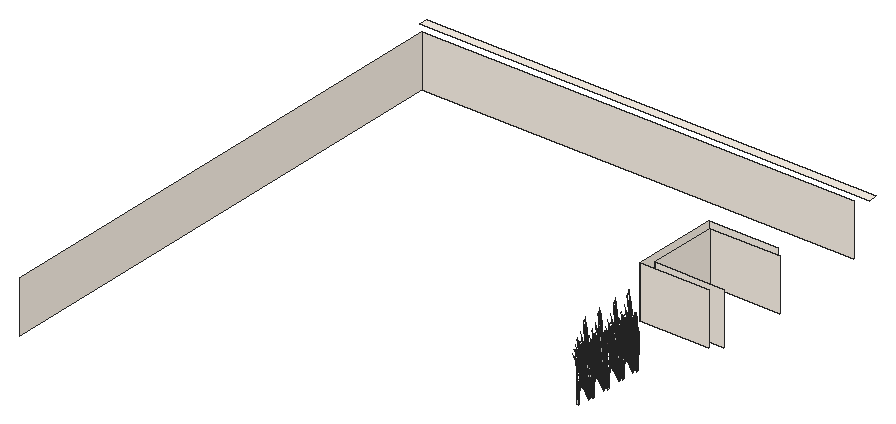
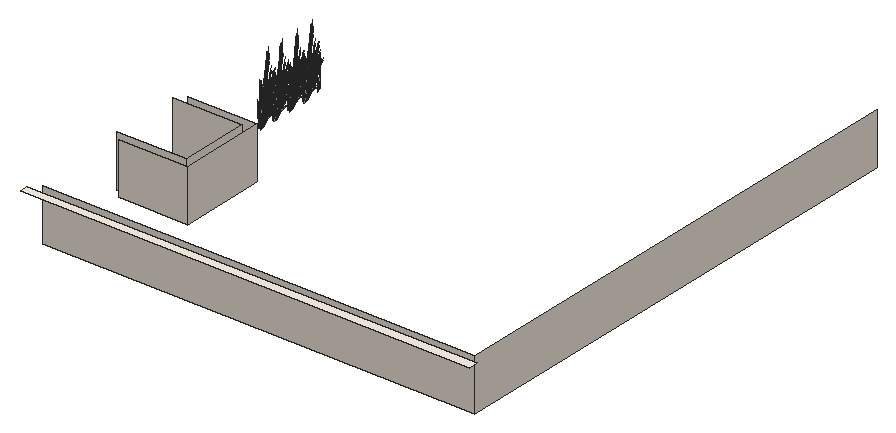
# SketchUp Ruby script. Lengths in inches.
U = 1.inch
M = Sketchup.active_model
def pt(a) = Geom::Point3d.new(a.map { |v| v * U })
def face(e, loops, mat)
  f = e.add_face(loops[0].map { |a| pt(a) })
  loops[1..].each { |l| e.add_face(l.map { |a| pt(a) }).erase! }
  f.material = f.back_material = mat if mat
  f
end
# faces: each face lists its corners as indices into pts; further lists are holes
def faces(e, pts, list, mat = nil) = list.each { |f| face(e, (f[0].is_a?(Array) ? f : [f]).map { |l| l.map { |i| pts[i] } }, mat) }
# xy, xz, yz: faces in a plane at the given z, y or x. An outline is a flat list of corners, or four numbers for a rectangle; further outlines are holes
def ring(l) = l.size == 4 ? [[l[0], l[1]], [l[2], l[1]], [l[2], l[3]], [l[0], l[3]]] : l.each_slice(2).to_a
def flat(e, list, mat, &to3) = list.each { |f| face(e, (f[0].is_a?(Array) ? f : [f]).map { |l| ring(l).map { |u, v| to3.(u, v) } }, mat) }
def xy(e, z, list, mat = nil) = flat(e, list, mat) { |x, y| [x, y, z] }
def xz(e, y, list, mat = nil) = flat(e, list, mat) { |x, z| [x, y, z] }
def yz(e, x, list, mat = nil) = flat(e, list, mat) { |y, z| [x, y, z] }
def lines(e, pts, list) = list.each { |a, b| e.add_line(pt(pts[a]), pt(pts[b])) }
# prism: a flat outline (further loops are holes) pulled along v
def prism(e, loops, v, mat = nil)
  f = face(e, loops, mat); d = Geom::Vector3d.new(v.map { |x| x * U })
  f.pushpull(f.normal.samedirection?(d) ? d.length : -d.length)
end
def box(e, o, s, mat = nil) = prism(e, [[o, [o[0] + s[0], o[1], o[2]], [o[0] + s[0], o[1] + s[1], o[2]], [o[0], o[1] + s[1], o[2]]]], [0, 0, s[2]], mat)
def at(x, y, z, deg = 0) = Geom::Transformation.translation(pt([x, y, z])) * Geom::Transformation.rotation(ORIGIN, Z_AXIS, deg.degrees)
def axes(o, x, y, z) = Geom::Transformation.new([*x, 0, *y, 0, *z, 0, *pt(o).to_a, 1])
def part(name) = M.definitions.add(name)
# library, detail: a bought-in or finely detailed component or shape, given as its bounding box
def library(name, o, s) = part(name).tap { |d| box(d.entities, o, s) }
def detail(e, o, s) = box(e.add_group.entities, o, s)
def put(e, d, t, mat = nil) = e.add_instance(d, t).tap { |i| i.material = mat if mat }
def group(e, t, mat = nil) = e.add_group.tap { |g| g.transformation = t; g.material = mat if mat }.entities
root = M.entities
M.materials.add("C01_Vanilla_Cream").color = [255, 246, 235]
M.materials.add("LightPink_Translucent").color = [144, 107, 117]
M.materials["LightPink_Translucent"].alpha = 0.75
c1 = part("blade")
p = [[2.15,0.21,22],[0,0.17,0],[0.09,0.45,0],[2.18,0.31,22],[2.29,0.31,22],[0.38,0.45,0],
  [2.48,0.24,33],[2.49,0.24,33],[2.48,0.22,33]]
faces(c1.entities,p,[[0,1,2,3],[4,5,2,3],[6,3,4,7],[8,0,3,6]])
c2 = part("seeds")
p = [[0.3,-0.1,1.38],[-0.01,-0.03,1.59],[-0.01,-0.03,0.03],[0.14,-0.07,-0.07],[0.29,-0.03,3],[0.15,0.01,3.11]]
faces(c2.entities,p,[[0,1,2,3],[1,0,4,5]],"LightPink_Translucent")
c3 = part("blade with seeds")
put(c3.entities,c1,at(0,0,0))
put(c3.entities,c2,axes([2.4,0.25,30.99],[1.5799,-0.05474,1.17369],[-0.12525,1.92788,0.29478],[-0.07173,-0.02425,1.56792]))
xy(root,690,[[48,366,360,372]],"C01_Vanilla_Cream")
xz(root,234,[[306,654,354,690]],"C01_Vanilla_Cream")
xz(root,240,[[312,654,360,690]],"C01_Vanilla_Cream")
xz(root,288,[[312,654,360,690]],"C01_Vanilla_Cream")
xz(root,294,[[306,654,354,690]],"C01_Vanilla_Cream")
xz(root,360,[[54,654,354,690]],"C01_Vanilla_Cream")
yz(root,54,[[12,654,360,690]],"C01_Vanilla_Cream")
yz(root,306,[[234,654,294,690]],"C01_Vanilla_Cream")
yz(root,312,[[240,654,288,690]],"C01_Vanilla_Cream")
put(root,c3,axes([339.83,148.68,657.18],[0.20495,-0.00938,1.40529],[-0.13596,0.40664,0.11363],[-0.29207,-0.02515,0.60075]))
put(root,c3,axes([339.83,161.3125,657.18],[0.20495,-0.00938,1.40529],[-0.13596,0.40664,0.11363],[-0.29207,-0.02515,0.60075]))
put(root,c3,axes([339.83,174.79,657.18],[0.20495,-0.00938,1.40529],[-0.13596,0.40664,0.11363],[-0.29207,-0.02515,0.60075]))
put(root,c3,axes([339.83,186.65,657.18],[0.20495,-0.00938,1.40529],[-0.13596,0.40664,0.11363],[-0.29207,-0.02515,0.60075]))
put(root,c3,axes([339.92,149.39,657.18],[0.17145,-0.08763,1.40529],[0.14434,0.4049,0.11363],[-0.26915,0.09151,0.60075]))
put(root,c3,axes([339.92,162.03,657.18],[0.17145,-0.08763,1.40529],[0.14434,0.4049,0.11363],[-0.26915,0.09151,0.60075]))
put(root,c3,axes([339.92,175.51,657.18],[0.17145,-0.08763,1.40529],[0.14434,0.4049,0.11363],[-0.26915,0.09151,0.60075]))
put(root,c3,axes([339.92,187.37,657.18],[0.17145,-0.08763,1.40529],[0.14434,0.4049,0.11363],[-0.26915,0.09151,0.60075]))
put(root,c3,axes([339.39,150.08,656.125],[0.17172,0.03401,1.17261],[0.11068,0.34736,-0.25218],[-0.23326,0.06502,0.50135]))
put(root,c3,axes([339.39,162.72,656.125],[0.17172,0.03401,1.17261],[0.11068,0.34736,-0.25218],[-0.23326,0.06502,0.50135]))
put(root,c3,axes([339.39,176.2,656.125],[0.17172,0.03401,1.17261],[0.11068,0.34736,-0.25218],[-0.23326,0.06502,0.50135]))
put(root,c3,axes([339.39,188.06,656.125],[0.17172,0.03401,1.17261],[0.11068,0.34736,-0.25218],[-0.23326,0.06502,0.50135]))
put(root,c3,axes([340.9,148.97,656.74],[0.14045,-0.05993,1.45192],[0.04843,0.41842,0.11363],[-0.30422,0.05552,0.51893]))
put(root,c3,axes([340.9,161.61,656.74],[0.14045,-0.05993,1.45192],[0.04843,0.41842,0.11363],[-0.30422,0.05552,0.51893]))
put(root,c3,axes([340.9,175.08,656.74],[0.14045,-0.05993,1.45192],[0.04843,0.41842,0.11363],[-0.30422,0.05552,0.51893]))
put(root,c3,axes([340.9,186.95,656.74],[0.14045,-0.05993,1.45192],[0.04843,0.41842,0.11363],[-0.30422,0.05552,0.51893]))
put(root,c3,axes([339.39,149.25,657.87],[-0.08069,0.05378,1.43454],[0.00686,0.39297,-0.22687],[-0.18495,0.0511,0.11505]))
put(root,c3,axes([339.39,161.89,657.87],[-0.08069,0.05378,1.43454],[0.00686,0.39297,-0.22687],[-0.18495,0.0511,0.11505]))
put(root,c3,axes([339.39,175.36,657.87],[-0.08069,0.05378,1.43454],[0.00686,0.39297,-0.22687],[-0.18495,0.0511,0.11505]))
put(root,c3,axes([339.39,187.23,657.87],[-0.08069,0.05378,1.43454],[0.00686,0.39297,-0.22687],[-0.18495,0.0511,0.11505]))
put(root,c3,axes([340.45,148.3,658.08],[-0.49394,-0.00997,-0.58257],[0.03317,-0.42002,0.0703],[-0.20925,-0.04433,0.8241]))
put(root,c3,axes([340.45,160.9375,658.08],[-0.49394,-0.00997,-0.58257],[0.03317,-0.42002,0.0703],[-0.20925,-0.04433,0.8241]))
put(root,c3,axes([340.45,174.41,658.08],[-0.49394,-0.00997,-0.58257],[0.03317,-0.42002,0.0703],[-0.20925,-0.04433,0.8241]))
put(root,c3,axes([340.45,186.27,658.08],[-0.49394,-0.00997,-0.58257],[0.03317,-0.42002,0.0703],[-0.20925,-0.04433,0.8241]))
put(root,c3,axes([340.05,148.4,656.125],[0.09647,0.11534,1.17261],[-0.2223,0.31351,-0.25218],[-0.22826,-0.07493,0.50135]))
put(root,c3,axes([340.05,161.04,656.125],[0.09647,0.11534,1.17261],[-0.2223,0.31351,-0.25218],[-0.22826,-0.07493,0.50135]))
put(root,c3,axes([340.05,174.52,656.125],[0.09647,0.11534,1.17261],[-0.2223,0.31351,-0.25218],[-0.22826,-0.07493,0.50135]))
put(root,c3,axes([340.05,186.375,656.125],[0.09647,0.11534,1.17261],[-0.2223,0.31351,-0.25218],[-0.22826,-0.07493,0.50135]))
put(root,c3,axes([339.65,149.03,657.71],[-0.41064,-0.11557,-0.29039],[0.11977,-0.33716,0.3749],[-0.16533,0.03092,0.71734]))
put(root,c3,axes([339.65,161.66,657.71],[-0.41064,-0.11557,-0.29039],[0.11977,-0.33716,0.3749],[-0.16533,0.03092,0.71734]))
put(root,c3,axes([339.65,175.14,657.71],[-0.41064,-0.11557,-0.29039],[0.11977,-0.33716,0.3749],[-0.16533,0.03092,0.71734]))
put(root,c3,axes([339.65,187,657.71],[-0.41064,-0.11557,-0.29039],[0.11977,-0.33716,0.3749],[-0.16533,0.03092,0.71734]))
put(root,c3,axes([340.22,148.02,657.18],[0.18354,0.07137,1.40529],[-0.37983,0.29943,0.11363],[-0.23673,-0.13508,0.60075]))
put(root,c3,axes([340.22,160.66,657.18],[0.18354,0.07137,1.40529],[-0.37983,0.29943,0.11363],[-0.23673,-0.13508,0.60075]))
put(root,c3,axes([340.22,174.14,657.18],[0.18354,0.07137,1.40529],[-0.37983,0.29943,0.11363],[-0.23673,-0.13508,0.60075]))
put(root,c3,axes([340.22,186,657.18],[0.18354,0.07137,1.40529],[-0.37983,0.29943,0.11363],[-0.23673,-0.13508,0.60075]))
put(root,c3,axes([338.5,149.65,657.86],[0.06306,0.01111,1.45454],[0.19508,0.36602,-0.13744],[-0.12909,0.09607,0.2574]))
put(root,c3,axes([338.5,162.28,657.86],[0.06306,0.01111,1.45454],[0.19508,0.36602,-0.13744],[-0.12909,0.09607,0.2574]))
put(root,c3,axes([338.5,175.76,657.86],[0.06306,0.01111,1.45454],[0.19508,0.36602,-0.13744],[-0.12909,0.09607,0.2574]))
put(root,c3,axes([338.5,187.625,657.86],[0.06306,0.01111,1.45454],[0.19508,0.36602,-0.13744],[-0.12909,0.09607,0.2574]))
put(root,c3,axes([339.94,149.2,657.84],[-0.13386,0.37682,-0.41901],[-0.45895,-0.12916,-0.32456],[-0.18478,0.03455,0.80174]))
put(root,c3,axes([339.94,161.84,657.84],[-0.13386,0.37682,-0.41901],[-0.45895,-0.12916,-0.32456],[-0.18478,0.03455,0.80174]))
put(root,c3,axes([339.94,175.3125,657.84],[-0.13386,0.37682,-0.41901],[-0.45895,-0.12916,-0.32456],[-0.18478,0.03455,0.80174]))
put(root,c3,axes([339.94,187.17,657.84],[-0.13386,0.37682,-0.41901],[-0.45895,-0.12916,-0.32456],[-0.18478,0.03455,0.80174]))
put(root,c3,axes([340.28,148.38,657.84],[-0.35879,0.27441,-0.41901],[-0.31422,-0.28988,-0.32456],[-0.18229,-0.04175,0.80174]))
put(root,c3,axes([340.28,161.02,657.84],[-0.35879,0.27441,-0.41901],[-0.31422,-0.28988,-0.32456],[-0.18229,-0.04175,0.80174]))
put(root,c3,axes([340.28,174.5,657.84],[-0.35879,0.27441,-0.41901],[-0.31422,-0.28988,-0.32456],[-0.18229,-0.04175,0.80174]))
put(root,c3,axes([340.28,186.36,657.84],[-0.35879,0.27441,-0.41901],[-0.31422,-0.28988,-0.32456],[-0.18229,-0.04175,0.80174]))
put(root,c3,axes([339.7,149.17,655.22],[0.01253,0.06529,1.44601],[-0.25262,0.34095,-0.2209],[-0.17944,-0.01719,0.2463]))
put(root,c3,axes([339.7,161.8125,655.22],[0.01253,0.06529,1.44601],[-0.25262,0.34095,-0.2209],[-0.17944,-0.01719,0.2463]))
put(root,c3,axes([339.7,175.29,655.22],[0.01253,0.06529,1.44601],[-0.25262,0.34095,-0.2209],[-0.17944,-0.01719,0.2463]))
put(root,c3,axes([339.7,187.15,655.22],[0.01253,0.06529,1.44601],[-0.25262,0.34095,-0.2209],[-0.17944,-0.01719,0.2463]))
put(root,c3,axes([339.78,147.61,657.86],[0.03663,0.04134,1.45454],[-0.17659,0.37163,-0.13744],[-0.17885,0.00269,0.2574]))
put(root,c3,axes([339.78,160.25,657.86],[0.03663,0.04134,1.45454],[-0.17659,0.37163,-0.13744],[-0.17885,0.00269,0.2574]))
put(root,c3,axes([339.78,173.73,657.86],[0.03663,0.04134,1.45454],[-0.17659,0.37163,-0.13744],[-0.17885,0.00269,0.2574]))
put(root,c3,axes([339.78,185.59,657.86],[0.03663,0.04134,1.45454],[-0.17659,0.37163,-0.13744],[-0.17885,0.00269,0.2574]))
put(root,c3,axes([339.03,150.81,656.27],[0.20592,-0.18775,0.94186],[0.08126,0.29723,0.69201],[-0.14881,0.05322,0.20745]))
put(root,c3,axes([339.03,163.45,656.27],[0.20592,-0.18775,0.94186],[0.08126,0.29723,0.69201],[-0.14881,0.05322,0.20745]))
put(root,c3,axes([339.03,176.92,656.27],[0.20592,-0.18775,0.94186],[0.08126,0.29723,0.69201],[-0.14881,0.05322,0.20745]))
put(root,c3,axes([339.03,188.79,656.27],[0.20592,-0.18775,0.94186],[0.08126,0.29723,0.69201],[-0.14881,0.05322,0.20745]))
put(root,c3,axes([340.1875,147.37,657.87],[-0.10632,-0.00292,1.43454],[-0.33847,0.29241,-0.22687],[-0.1806,-0.05975,0.11505]))
put(root,c3,axes([340.1875,160,657.87],[-0.10632,-0.00292,1.43454],[-0.33847,0.29241,-0.22687],[-0.1806,-0.05975,0.11505]))
put(root,c3,axes([340.1875,173.48,657.87],[-0.10632,-0.00292,1.43454],[-0.33847,0.29241,-0.22687],[-0.1806,-0.05975,0.11505]))
put(root,c3,axes([340.1875,185.34,657.87],[-0.10632,-0.00292,1.43454],[-0.33847,0.29241,-0.22687],[-0.1806,-0.05975,0.11505]))
put(root,c3,axes([339.75,148.98,657.88],[0.1396,-0.37772,0.39362],[0.45895,0.12916,0.32456],[-0.18049,0.0227,0.8145]))
put(root,c3,axes([339.75,161.62,657.88],[0.1396,-0.37772,0.39362],[0.45895,0.12916,0.32456],[-0.18049,0.0227,0.8145]))
put(root,c3,axes([339.75,175.1,657.88],[0.1396,-0.37772,0.39362],[0.45895,0.12916,0.32456],[-0.18049,0.0227,0.8145]))
put(root,c3,axes([339.75,186.96,657.88],[0.1396,-0.37772,0.39362],[0.45895,0.12916,0.32456],[-0.18049,0.0227,0.8145]))
put(root,c3,axes([339.91,148.875,658.13],[0.24861,0.37512,-0.09971],[-0.44125,0.18434,-0.55346],[-0.18594,0.04949,0.84097]))
put(root,c3,axes([339.91,161.51,658.13],[0.24861,0.37512,-0.09971],[-0.44125,0.18434,-0.55346],[-0.18594,0.04949,0.84097]))
put(root,c3,axes([339.91,174.99,658.13],[0.24861,0.37512,-0.09971],[-0.44125,0.18434,-0.55346],[-0.18594,0.04949,0.84097]))
put(root,c3,axes([339.91,186.85,658.13],[0.24861,0.37512,-0.09971],[-0.44125,0.18434,-0.55346],[-0.18594,0.04949,0.84097]))
put(root,c3,axes([340.47,148.1,658.13],[-0.02646,0.4213,-0.09971],[-0.50094,-0.01152,-0.55346],[-0.19293,-0.02926,0.84097]))
put(root,c3,axes([340.47,160.73,658.13],[-0.02646,0.4213,-0.09971],[-0.50094,-0.01152,-0.55346],[-0.19293,-0.02926,0.84097]))
put(root,c3,axes([340.47,174.21,658.13],[-0.02646,0.4213,-0.09971],[-0.50094,-0.01152,-0.55346],[-0.19293,-0.02926,0.84097]))
put(root,c3,axes([340.47,186.07,658.13],[-0.02646,0.4213,-0.09971],[-0.50094,-0.01152,-0.55346],[-0.19293,-0.02926,0.84097]))
put(root,c3,axes([340.15,148.125,657.71],[-0.28114,-0.25937,-0.29039],[0.32102,-0.24553,0.3749],[-0.16311,-0.03736,0.71734]))
put(root,c3,axes([340.15,160.76,657.71],[-0.28114,-0.25937,-0.29039],[0.32102,-0.24553,0.3749],[-0.16311,-0.03736,0.71734]))
put(root,c3,axes([340.15,174.24,657.71],[-0.28114,-0.25937,-0.29039],[0.32102,-0.24553,0.3749],[-0.16311,-0.03736,0.71734]))
put(root,c3,axes([340.15,186.1,657.71],[-0.28114,-0.25937,-0.29039],[0.32102,-0.24553,0.3749],[-0.16311,-0.03736,0.71734]))
put(root,c3,axes([339.71,148.88,657.88],[-0.18148,-0.28246,0.05273],[0.33093,-0.13825,0.41509],[-0.14588,0.02728,0.63295]))
put(root,c3,axes([339.71,161.52,657.88],[-0.18148,-0.28246,0.05273],[0.33093,-0.13825,0.41509],[-0.14588,0.02728,0.63295]))
put(root,c3,axes([339.71,175,657.88],[-0.18148,-0.28246,0.05273],[0.33093,-0.13825,0.41509],[-0.14588,0.02728,0.63295]))
put(root,c3,axes([339.71,186.86,657.88],[-0.18148,-0.28246,0.05273],[0.33093,-0.13825,0.41509],[-0.14588,0.02728,0.63295]))
put(root,c3,axes([340.55,149.66,657.18],[0.12341,-0.12729,1.40529],[0.31162,0.34357,0.11363],[-0.21373,0.15646,0.60075]))
put(root,c3,axes([340.55,162.3,657.18],[0.12341,-0.12729,1.40529],[0.31162,0.34357,0.11363],[-0.21373,0.15646,0.60075]))
put(root,c3,axes([340.55,175.78,657.18],[0.12341,-0.12729,1.40529],[0.31162,0.34357,0.11363],[-0.21373,0.15646,0.60075]))
put(root,c3,axes([340.55,187.64,657.18],[0.12341,-0.12729,1.40529],[0.31162,0.34357,0.11363],[-0.21373,0.15646,0.60075]))
put(root,c3,axes([339.8,150,657.71],[-0.43011,0.0592,-0.29039],[-0.11357,-0.33844,0.3749],[-0.12326,0.0909,0.71734]))
put(root,c3,axes([339.8,162.64,657.71],[-0.43011,0.0592,-0.29039],[-0.11357,-0.33844,0.3749],[-0.12326,0.0909,0.71734]))
put(root,c3,axes([339.8,176.11,657.71],[-0.43011,0.0592,-0.29039],[-0.11357,-0.33844,0.3749],[-0.12326,0.0909,0.71734]))
put(root,c3,axes([339.8,187.97,657.71],[-0.43011,0.0592,-0.29039],[-0.11357,-0.33844,0.3749],[-0.12326,0.0909,0.71734]))
put(root,c3,axes([339.57,151,655.22],[0.06628,0.04139,1.44601],[0.11238,0.38347,-0.2209],[-0.14689,0.08177,0.2463]))
put(root,c3,axes([339.57,163.64,655.22],[0.06628,0.04139,1.44601],[0.11238,0.38347,-0.2209],[-0.14689,0.08177,0.2463]))
put(root,c3,axes([339.57,177.12,655.22],[0.06628,0.04139,1.44601],[0.11238,0.38347,-0.2209],[-0.14689,0.08177,0.2463]))
put(root,c3,axes([339.57,188.98,655.22],[0.06628,0.04139,1.44601],[0.11238,0.38347,-0.2209],[-0.14689,0.08177,0.2463]))
put(root,c3,axes([339.47,148.75,656.27],[0.31546,-0.02964,0.94186],[-0.20011,0.26119,0.69201],[-0.15589,-0.03918,0.20745]))
put(root,c3,axes([339.47,161.38,656.27],[0.31546,-0.02964,0.94186],[-0.20011,0.26119,0.69201],[-0.15589,-0.03918,0.20745]))
put(root,c3,axes([339.47,174.86,656.27],[0.31546,-0.02964,0.94186],[-0.20011,0.26119,0.69201],[-0.15589,-0.03918,0.20745]))
put(root,c3,axes([339.47,186.72,656.27],[0.31546,-0.02964,0.94186],[-0.20011,0.26119,0.69201],[-0.15589,-0.03918,0.20745]))
put(root,c3,axes([339.86,149.92,657.88],[-0.12254,-0.38127,0.39362],[0.48071,-0.06617,0.32456],[-0.14168,0.08967,0.8145]))
put(root,c3,axes([339.86,162.5625,657.88],[-0.12254,-0.38127,0.39362],[0.48071,-0.06617,0.32456],[-0.14168,0.08967,0.8145]))
put(root,c3,axes([339.86,176.04,657.88],[-0.12254,-0.38127,0.39362],[0.48071,-0.06617,0.32456],[-0.14168,0.08967,0.8145]))
put(root,c3,axes([339.86,187.9,657.88],[-0.12254,-0.38127,0.39362],[0.48071,-0.06617,0.32456],[-0.14168,0.08967,0.8145]))
put(root,c3,axes([340.11,148.03,658.18],[0.40806,-0.30572,0.44086],[0.35193,0.32467,0.3635],[-0.19145,-0.05639,0.91224]))
put(root,c3,axes([340.11,160.67,658.18],[0.40806,-0.30572,0.44086],[0.35193,0.32467,0.3635],[-0.19145,-0.05639,0.91224]))
put(root,c3,axes([340.11,174.14,658.18],[0.40806,-0.30572,0.44086],[0.35193,0.32467,0.3635],[-0.19145,-0.05639,0.91224]))
put(root,c3,axes([340.11,186,658.18],[0.40806,-0.30572,0.44086],[0.35193,0.32467,0.3635],[-0.19145,-0.05639,0.91224]))
put(root,c3,axes([339.76,149.85,657.88],[-0.33921,-0.17422,0.05273],[0.19749,-0.2481,0.41509],[-0.10876,0.08021,0.63295]))
put(root,c3,axes([339.76,162.49,657.88],[-0.33921,-0.17422,0.05273],[0.19749,-0.2481,0.41509],[-0.10876,0.08021,0.63295]))
put(root,c3,axes([339.76,175.97,657.88],[-0.33921,-0.17422,0.05273],[0.19749,-0.2481,0.41509],[-0.10876,0.08021,0.63295]))
put(root,c3,axes([339.76,187.83,657.88],[-0.33921,-0.17422,0.05273],[0.19749,-0.2481,0.41509],[-0.10876,0.08021,0.63295]))
put(root,c3,axes([340.45,136.89,657.18],[0.092,-0.14239,1.40529],[0.38596,0.29467,0.11363],[-0.17411,0.18366,0.60075]))
put(root,c3,axes([340.45,149.98,657.18],[0.092,-0.14239,1.40529],[0.38596,0.29467,0.11363],[-0.17411,0.18366,0.60075]))
put(root,c3,axes([340.45,162.62,657.18],[0.092,-0.14239,1.40529],[0.38596,0.29467,0.11363],[-0.17411,0.18366,0.60075]))
put(root,c3,axes([340.45,176.09,657.18],[0.092,-0.14239,1.40529],[0.38596,0.29467,0.11363],[-0.17411,0.18366,0.60075]))
put(root,c3,axes([340.45,187.95,657.18],[0.092,-0.14239,1.40529],[0.38596,0.29467,0.11363],[-0.17411,0.18366,0.60075]))
put(root,c3,axes([340.09,148.99,658.14],[0.41064,0.11557,0.29039],[-0.11977,0.33716,-0.3749],[-0.16533,0.03092,0.71734]))
put(root,c3,axes([340.09,161.625,658.14],[0.41064,0.11557,0.29039],[-0.11977,0.33716,-0.3749],[-0.16533,0.03092,0.71734]))
put(root,c3,axes([340.09,175.1,658.14],[0.41064,0.11557,0.29039],[-0.11977,0.33716,-0.3749],[-0.16533,0.03092,0.71734]))
put(root,c3,axes([340.09,186.96,658.14],[0.41064,0.11557,0.29039],[-0.11977,0.33716,-0.3749],[-0.16533,0.03092,0.71734]))
put(root,c3,axes([340.16,150.04,657.84],[0.12693,0.37826,-0.41901],[-0.48071,0.06617,-0.32456],[-0.13776,0.1016,0.80174]))
put(root,c3,axes([340.16,162.67,657.84],[0.12693,0.37826,-0.41901],[-0.48071,0.06617,-0.32456],[-0.13776,0.1016,0.80174]))
put(root,c3,axes([340.16,176.15,657.84],[0.12693,0.37826,-0.41901],[-0.48071,0.06617,-0.32456],[-0.13776,0.1016,0.80174]))
put(root,c3,axes([340.16,188.01,657.84],[0.12693,0.37826,-0.41901],[-0.48071,0.06617,-0.32456],[-0.13776,0.1016,0.80174]))
put(root,c3,axes([340.29,148.03,657.88],[0.02488,-0.31501,0.05273],[0.3757,0.00864,0.41509],[-0.14392,-0.03296,0.63295]))
put(root,c3,axes([340.29,160.66,657.88],[0.02488,-0.31501,0.05273],[0.3757,0.00864,0.41509],[-0.14392,-0.03296,0.63295]))
put(root,c3,axes([340.29,174.14,657.88],[0.02488,-0.31501,0.05273],[0.3757,0.00864,0.41509],[-0.14392,-0.03296,0.63295]))
put(root,c3,axes([340.29,186,657.88],[0.02488,-0.31501,0.05273],[0.3757,0.00864,0.41509],[-0.14392,-0.03296,0.63295]))
put(root,c3,axes([339.41,137.625,657.87],[-0.01228,0.08198,1.43454],[0.34856,0.28519,-0.22687],[-0.09125,0.13486,0.11505]))
put(root,c3,axes([339.41,150.72,657.87],[-0.01228,0.08198,1.43454],[0.34856,0.28519,-0.22687],[-0.09125,0.13486,0.11505]))
put(root,c3,axes([339.41,163.35,657.87],[-0.01228,0.08198,1.43454],[0.34856,0.28519,-0.22687],[-0.09125,0.13486,0.11505]))
put(root,c3,axes([339.41,176.83,657.87],[-0.01228,0.08198,1.43454],[0.34856,0.28519,-0.22687],[-0.09125,0.13486,0.11505]))
put(root,c3,axes([339.41,188.69,657.87],[-0.01228,0.08198,1.43454],[0.34856,0.28519,-0.22687],[-0.09125,0.13486,0.11505]))
put(root,c3,axes([341.36,149.77,655.6875],[-0.514,-0.06792,-0.51129],[0.10846,-0.41895,-0.13419],[-0.15339,-0.05076,1.12859]))
put(root,c3,axes([341.36,162.4,655.6875],[-0.514,-0.06792,-0.51129],[0.10846,-0.41895,-0.13419],[-0.15339,-0.05076,1.12859]))
put(root,c3,axes([341.36,175.88,655.6875],[-0.514,-0.06792,-0.51129],[0.10846,-0.41895,-0.13419],[-0.15339,-0.05076,1.12859]))
put(root,c3,axes([341.36,187.74,655.6875],[-0.514,-0.06792,-0.51129],[0.10846,-0.41895,-0.13419],[-0.15339,-0.05076,1.12859]))
put(root,c3,axes([341.45,147.48,658.45],[-0.32977,0.39714,-0.11168],[-0.47757,-0.2288,-0.61987],[-0.16601,-0.1122,0.94188]))
put(root,c3,axes([341.45,160.12,658.45],[-0.32977,0.39714,-0.11168],[-0.47757,-0.2288,-0.61987],[-0.16601,-0.1122,0.94188]))
put(root,c3,axes([341.45,173.6,658.45],[-0.32977,0.39714,-0.11168],[-0.47757,-0.2288,-0.61987],[-0.16601,-0.1122,0.94188]))
put(root,c3,axes([341.45,185.46,658.45],[-0.32977,0.39714,-0.11168],[-0.47757,-0.2288,-0.61987],[-0.16601,-0.1122,0.94188]))
put(root,c3,axes([340.55,148.26,658.14],[0.28114,0.25937,0.29039],[-0.32102,0.24553,-0.3749],[-0.16311,-0.03736,0.71734]))
put(root,c3,axes([340.55,160.9,658.14],[0.28114,0.25937,0.29039],[-0.32102,0.24553,-0.3749],[-0.16311,-0.03736,0.71734]))
put(root,c3,axes([340.55,174.375,658.14],[0.28114,0.25937,0.29039],[-0.32102,0.24553,-0.3749],[-0.16311,-0.03736,0.71734]))
put(root,c3,axes([340.55,186.24,658.14],[0.28114,0.25937,0.29039],[-0.32102,0.24553,-0.3749],[-0.16311,-0.03736,0.71734]))
put(root,c3,axes([341.31,147.8,658.08],[-0.42133,-0.20023,-0.58257],[0.29943,-0.35088,0.0703],[-0.15265,-0.11956,0.8241]))
put(root,c3,axes([341.31,160.44,658.08],[-0.42133,-0.20023,-0.58257],[0.29943,-0.35088,0.0703],[-0.15265,-0.11956,0.8241]))
put(root,c3,axes([341.31,173.92,658.08],[-0.42133,-0.20023,-0.58257],[0.29943,-0.35088,0.0703],[-0.15265,-0.11956,0.8241]))
put(root,c3,axes([341.31,185.78,658.08],[-0.42133,-0.20023,-0.58257],[0.29943,-0.35088,0.0703],[-0.15265,-0.11956,0.8241]))
put(root,c3,axes([341.11,147.8125,657.84],[-0.48758,0.09847,-0.41901],[-0.08529,-0.37293,-0.32456],[-0.13096,-0.10687,0.80174]))
put(root,c3,axes([341.11,160.45,657.84],[-0.48758,0.09847,-0.41901],[-0.08529,-0.37293,-0.32456],[-0.13096,-0.10687,0.80174]))
put(root,c3,axes([341.11,173.93,657.84],[-0.48758,0.09847,-0.41901],[-0.08529,-0.37293,-0.32456],[-0.13096,-0.10687,0.80174]))
put(root,c3,axes([341.11,185.79,657.84],[-0.48758,0.09847,-0.41901],[-0.08529,-0.37293,-0.32456],[-0.13096,-0.10687,0.80174]))
put(root,c3,axes([340.68,150.56,655.65],[-0.46245,-0.20713,-0.40713],[0.27641,-0.37142,0],[-0.10533,-0.04718,1.29153]))
put(root,c3,axes([340.68,163.2,655.65],[-0.46245,-0.20713,-0.40713],[0.27641,-0.37142,0],[-0.10533,-0.04718,1.29153]))
put(root,c3,axes([340.68,176.67,655.65],[-0.46245,-0.20713,-0.40713],[0.27641,-0.37142,0],[-0.10533,-0.04718,1.29153]))
put(root,c3,axes([340.68,188.54,655.65],[-0.46245,-0.20713,-0.40713],[0.27641,-0.37142,0],[-0.10533,-0.04718,1.29153]))
put(root,c3,axes([340.48,147.47,655.22],[-0.04786,0.05457,1.44601],[-0.48369,0.11766,-0.2209],[-0.11685,-0.10703,0.2463]))
put(root,c3,axes([340.48,160.11,655.22],[-0.04786,0.05457,1.44601],[-0.48369,0.11766,-0.2209],[-0.11685,-0.10703,0.2463]))
put(root,c3,axes([340.48,173.59,655.22],[-0.04786,0.05457,1.44601],[-0.48369,0.11766,-0.2209],[-0.11685,-0.10703,0.2463]))
put(root,c3,axes([340.48,185.45,655.22],[-0.04786,0.05457,1.44601],[-0.48369,0.11766,-0.2209],[-0.11685,-0.10703,0.2463]))
put(root,c3,axes([339.93,149.77,658.13],[0.45707,0.22842,-0.09971],[-0.26332,0.3308,-0.55346],[-0.12913,0.11499,0.84097]))
put(root,c3,axes([339.93,162.4,658.13],[0.45707,0.22842,-0.09971],[-0.26332,0.3308,-0.55346],[-0.12913,0.11499,0.84097]))
put(root,c3,axes([339.93,175.88,658.13],[0.45707,0.22842,-0.09971],[-0.26332,0.3308,-0.55346],[-0.12913,0.11499,0.84097]))
put(root,c3,axes([339.93,187.74,658.13],[0.45707,0.22842,-0.09971],[-0.26332,0.3308,-0.55346],[-0.12913,0.11499,0.84097]))
put(root,c3,axes([340.96,150.81,655.95],[-0.30893,0.41511,0],[-0.51685,-0.2315,-0.42318],[-0.11772,-0.05273,1.34243]))
put(root,c3,axes([340.96,163.45,655.95],[-0.30893,0.41511,0],[-0.51685,-0.2315,-0.42318],[-0.11772,-0.05273,1.34243]))
put(root,c3,axes([340.96,176.92,655.95],[-0.30893,0.41511,0],[-0.51685,-0.2315,-0.42318],[-0.11772,-0.05273,1.34243]))
put(root,c3,axes([340.96,188.79,655.95],[-0.30893,0.41511,0],[-0.51685,-0.2315,-0.42318],[-0.11772,-0.05273,1.34243]))
put(root,c3,axes([339.18,150.76,658.63],[0.43603,0.11058,-0.0532],[-0.13413,0.34034,-0.24121],[-0.07132,0.05167,0.7956]))
put(root,c3,axes([339.18,163.4,658.63],[0.43603,0.11058,-0.0532],[-0.13413,0.34034,-0.24121],[-0.07132,0.05167,0.7956]))
put(root,c3,axes([339.18,176.875,658.63],[0.43603,0.11058,-0.0532],[-0.13413,0.34034,-0.24121],[-0.07132,0.05167,0.7956]))
put(root,c3,axes([339.18,188.73,658.63],[0.43603,0.11058,-0.0532],[-0.13413,0.34034,-0.24121],[-0.07132,0.05167,0.7956]))
put(root,c3,axes([340.15,149.8,658.14],[0.43011,-0.0592,0.29039],[0.11357,0.33844,-0.3749],[-0.12326,0.0909,0.71734]))
put(root,c3,axes([340.15,162.44,658.14],[0.43011,-0.0592,0.29039],[0.11357,0.33844,-0.3749],[-0.12326,0.0909,0.71734]))
put(root,c3,axes([340.15,175.91,658.14],[0.43011,-0.0592,0.29039],[0.11357,0.33844,-0.3749],[-0.12326,0.0909,0.71734]))
put(root,c3,axes([340.15,187.77,658.14],[0.43011,-0.0592,0.29039],[0.11357,0.33844,-0.3749],[-0.12326,0.0909,0.71734]))
put(root,c3,axes([340.4,138.32,656.125],[0.15593,-0.06535,1.17261],[0.38498,0.19705,-0.25218],[-0.11459,0.1705,0.50135]))
put(root,c3,axes([340.4,151.41,656.125],[0.15593,-0.06535,1.17261],[0.38498,0.19705,-0.25218],[-0.11459,0.1705,0.50135]))
put(root,c3,axes([340.4,164.05,656.125],[0.15593,-0.06535,1.17261],[0.38498,0.19705,-0.25218],[-0.11459,0.1705,0.50135]))
put(root,c3,axes([340.4,177.52,656.125],[0.15593,-0.06535,1.17261],[0.38498,0.19705,-0.25218],[-0.11459,0.1705,0.50135]))
put(root,c3,axes([340.4,189.39,656.125],[0.15593,-0.06535,1.17261],[0.38498,0.19705,-0.25218],[-0.11459,0.1705,0.50135]))
put(root,c3,axes([340.18,147.68,655.74],[-0.14254,0.33827,-0.03192],[-0.4387,-0.10405,-0.14473],[-0.06661,-0.05533,0.47736]))
put(root,c3,axes([340.18,160.32,655.74],[-0.14254,0.33827,-0.03192],[-0.4387,-0.10405,-0.14473],[-0.06661,-0.05533,0.47736]))
put(root,c3,axes([340.18,173.8,655.74],[-0.14254,0.33827,-0.03192],[-0.4387,-0.10405,-0.14473],[-0.06661,-0.05533,0.47736]))
put(root,c3,axes([340.18,185.66,655.74],[-0.14254,0.33827,-0.03192],[-0.4387,-0.10405,-0.14473],[-0.06661,-0.05533,0.47736]))
put(root,c3,axes([341.32,146.54,657.86],[-0.00922,0.04965,1.45454],[-0.45464,0.18021,-0.13744],[-0.13379,-0.09212,0.2574]))
put(root,c3,axes([341.32,159.17,657.86],[-0.00922,0.04965,1.45454],[-0.45464,0.18021,-0.13744],[-0.13379,-0.09212,0.2574]))
put(root,c3,axes([341.32,172.65,657.86],[-0.00922,0.04965,1.45454],[-0.45464,0.18021,-0.13744],[-0.13379,-0.09212,0.2574]))
put(root,c3,axes([341.32,184.51,657.86],[-0.00922,0.04965,1.45454],[-0.45464,0.18021,-0.13744],[-0.13379,-0.09212,0.2574]))
put(root,c3,axes([340.83,147.26,656.125],[-0.02992,0.13552,1.17261],[-0.43742,0.11344,-0.25218],[-0.10225,-0.17516,0.50135]))
put(root,c3,axes([340.83,159.9,656.125],[-0.02992,0.13552,1.17261],[-0.43742,0.11344,-0.25218],[-0.10225,-0.17516,0.50135]))
put(root,c3,axes([340.83,173.37,656.125],[-0.02992,0.13552,1.17261],[-0.43742,0.11344,-0.25218],[-0.10225,-0.17516,0.50135]))
put(root,c3,axes([340.83,185.23,656.125],[-0.02992,0.13552,1.17261],[-0.43742,0.11344,-0.25218],[-0.10225,-0.17516,0.50135]))
put(root,c3,axes([340.98,147.61,657.18],[0.11295,0.13301,1.40529],[-0.52192,0.11198,0.11363],[-0.11796,-0.20881,0.60075]))
put(root,c3,axes([340.98,160.25,657.18],[0.11295,0.13301,1.40529],[-0.52192,0.11198,0.11363],[-0.11796,-0.20881,0.60075]))
put(root,c3,axes([340.98,173.72,657.18],[0.11295,0.13301,1.40529],[-0.52192,0.11198,0.11363],[-0.11796,-0.20881,0.60075]))
put(root,c3,axes([340.98,185.58,657.18],[0.11295,0.13301,1.40529],[-0.52192,0.11198,0.11363],[-0.11796,-0.20881,0.60075]))
put(root,c3,axes([341.94,149.83,656.1875],[-0.49889,0.27503,-0.23858],[-0.33175,-0.38862,-0.41002],[-0.12309,-0.03947,1.3096]))
put(root,c3,axes([341.94,162.47,656.1875],[-0.49889,0.27503,-0.23858],[-0.33175,-0.38862,-0.41002],[-0.12309,-0.03947,1.3096]))
put(root,c3,axes([341.94,175.94,656.1875],[-0.49889,0.27503,-0.23858],[-0.33175,-0.38862,-0.41002],[-0.12309,-0.03947,1.3096]))
put(root,c3,axes([341.94,187.8,656.1875],[-0.49889,0.27503,-0.23858],[-0.33175,-0.38862,-0.41002],[-0.12309,-0.03947,1.3096]))
put(root,c3,axes([340.5625,150.7,657.88],[-0.35185,-0.28265,0.39362],[0.37366,-0.24377,0.32456],[-0.0649,0.13261,0.8145]))
put(root,c3,axes([340.5625,163.33,657.88],[-0.35185,-0.28265,0.39362],[0.37366,-0.24377,0.32456],[-0.0649,0.13261,0.8145]))
put(root,c3,axes([340.5625,176.8125,657.88],[-0.35185,-0.28265,0.39362],[0.37366,-0.24377,0.32456],[-0.0649,0.13261,0.8145]))
put(root,c3,axes([340.5625,188.67,657.88],[-0.35185,-0.28265,0.39362],[0.37366,-0.24377,0.32456],[-0.0649,0.13261,0.8145]))
put(root,c3,axes([341.16,147.54,657.71],[-0.07631,-0.33368,-0.29039],[0.43626,-0.08811,0.3749],[-0.11718,-0.09562,0.71734]))
put(root,c3,axes([341.16,160.18,657.71],[-0.07631,-0.33368,-0.29039],[0.43626,-0.08811,0.3749],[-0.11718,-0.09562,0.71734]))
put(root,c3,axes([341.16,173.65,657.71],[-0.07631,-0.33368,-0.29039],[0.43626,-0.08811,0.3749],[-0.11718,-0.09562,0.71734]))
put(root,c3,axes([341.16,185.51,657.71],[-0.07631,-0.33368,-0.29039],[0.43626,-0.08811,0.3749],[-0.11718,-0.09562,0.71734]))
put(root,c3,axes([339.94,149.23,655.95],[-0.61786,0,0],[0,-0.463,-0.42318],[0,-0.10545,1.34243]))
put(root,c3,axes([339.94,161.87,655.95],[-0.61786,0,0],[0,-0.463,-0.42318],[0,-0.10545,1.34243]))
put(root,c3,axes([339.94,175.34,655.95],[-0.61786,0,0],[0,-0.463,-0.42318],[0,-0.10545,1.34243]))
put(root,c3,axes([339.94,187.2,655.95],[-0.61786,0,0],[0,-0.463,-0.42318],[0,-0.10545,1.34243]))
put(root,c3,axes([340.8125,150.4,655.66],[-0.11607,-0.36097,-0.25402],[0.46099,-0.1025,0.25402],[-0.09293,-0.04163,1.13959]))
put(root,c3,axes([340.8125,163.04,655.66],[-0.11607,-0.36097,-0.25402],[0.46099,-0.1025,0.25402],[-0.09293,-0.04163,1.13959]))
put(root,c3,axes([340.8125,176.52,655.66],[-0.11607,-0.36097,-0.25402],[0.46099,-0.1025,0.25402],[-0.09293,-0.04163,1.13959]))
put(root,c3,axes([340.8125,188.38,655.66],[-0.11607,-0.36097,-0.25402],[0.46099,-0.1025,0.25402],[-0.09293,-0.04163,1.13959]))
